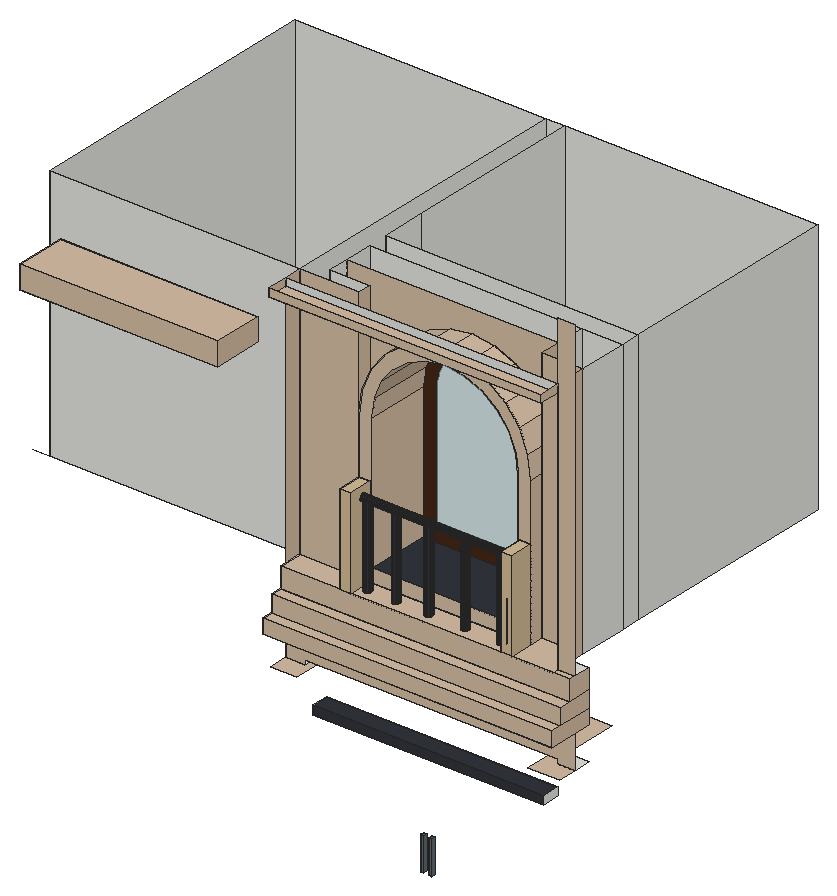
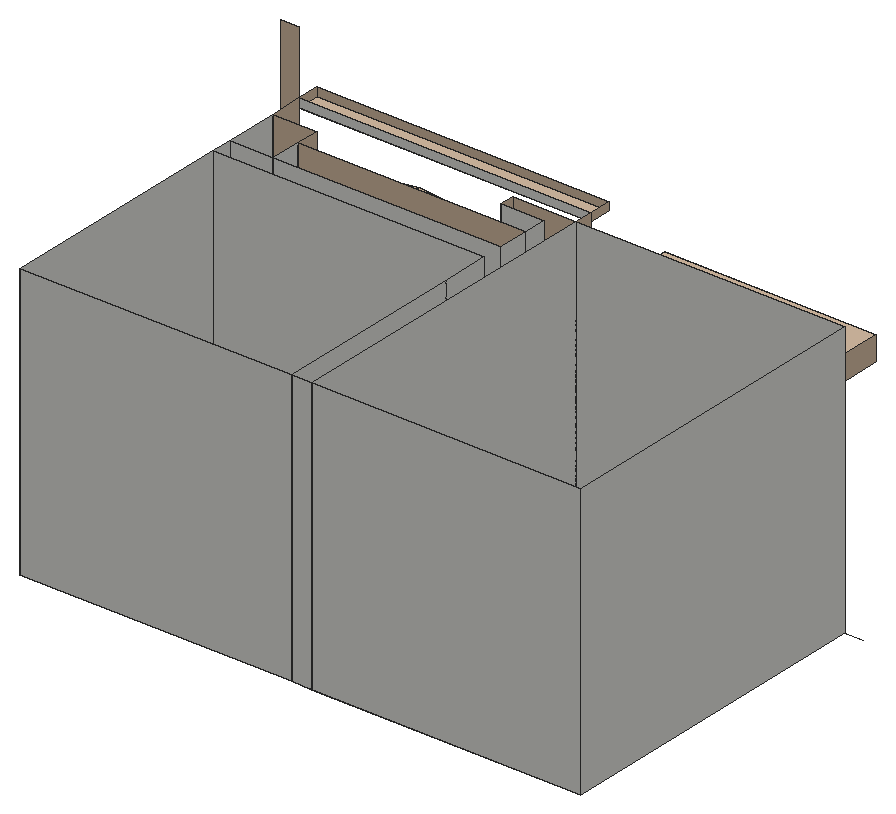
# SketchUp Ruby script. Lengths in inches.
U = 1.inch
M = Sketchup.active_model
def pt(a) = Geom::Point3d.new(a.map { |v| v * U })
def face(e, loops, mat)
  f = e.add_face(loops[0].map { |a| pt(a) })
  loops[1..].each { |l| e.add_face(l.map { |a| pt(a) }).erase! }
  f.material = f.back_material = mat if mat
  f
end
# faces: each face lists its corners as indices into pts; further lists are holes
def faces(e, pts, list, mat = nil) = list.each { |f| face(e, (f[0].is_a?(Array) ? f : [f]).map { |l| l.map { |i| pts[i] } }, mat) }
# xy, xz, yz: faces in a plane at the given z, y or x. An outline is a flat list of corners, or four numbers for a rectangle; further outlines are holes
def ring(l) = l.size == 4 ? [[l[0], l[1]], [l[2], l[1]], [l[2], l[3]], [l[0], l[3]]] : l.each_slice(2).to_a
def flat(e, list, mat, &to3) = list.each { |f| face(e, (f[0].is_a?(Array) ? f : [f]).map { |l| ring(l).map { |u, v| to3.(u, v) } }, mat) }
def xy(e, z, list, mat = nil) = flat(e, list, mat) { |x, y| [x, y, z] }
def xz(e, y, list, mat = nil) = flat(e, list, mat) { |x, z| [x, y, z] }
def yz(e, x, list, mat = nil) = flat(e, list, mat) { |y, z| [x, y, z] }
def lines(e, pts, list) = list.each { |a, b| e.add_line(pt(pts[a]), pt(pts[b])) }
# prism: a flat outline (further loops are holes) pulled along v
def prism(e, loops, v, mat = nil)
  f = face(e, loops, mat); d = Geom::Vector3d.new(v.map { |x| x * U })
  f.pushpull(f.normal.samedirection?(d) ? d.length : -d.length)
end
def box(e, o, s, mat = nil) = prism(e, [[o, [o[0] + s[0], o[1], o[2]], [o[0] + s[0], o[1] + s[1], o[2]], [o[0], o[1] + s[1], o[2]]]], [0, 0, s[2]], mat)
def at(x, y, z, deg = 0) = Geom::Transformation.translation(pt([x, y, z])) * Geom::Transformation.rotation(ORIGIN, Z_AXIS, deg.degrees)
def axes(o, x, y, z) = Geom::Transformation.new([*x, 0, *y, 0, *z, 0, *pt(o).to_a, 1])
def part(name) = M.definitions.add(name)
# library, detail: a bought-in or finely detailed component or shape, given as its bounding box
def library(name, o, s) = part(name).tap { |d| box(d.entities, o, s) }
def detail(e, o, s) = box(e.add_group.entities, o, s)
def put(e, d, t, mat = nil) = e.add_instance(d, t).tap { |i| i.material = mat if mat }
def group(e, t, mat = nil) = e.add_group.tap { |g| g.transformation = t; g.material = mat if mat }.entities
root = M.entities
M.materials.add("[Formica Beige]").color = [211, 187, 149]
M.materials.add("[Formica Laminate Dark]").color = [50, 53, 60]
M.materials.add("[Formica Laminate Light]").color = [213, 189, 164]
M.materials.add("[Formica Speckled Grey]").color = [94, 105, 111]
M.materials.add("[Translucent Glass Safety]").color = [204, 235, 244]
M.materials["[Translucent Glass Safety]"].alpha = 0.5
M.materials.add("[Wood Veneer 01]").color = [68, 40, 21]
xy(root,44.27,[[216.72,67.98,217.85,69.35],[219.85,67.98,220.97,69.35]],"[Formica Speckled Grey]")
xy(root,56.83,[[216.72,67.98,217.85,69.35],[219.85,67.98,220.97,69.35]],"[Formica Speckled Grey]")
xy(root,81.84,[[[175.36,69.35,216.21,75.87],[213.5,71.93,213.76,71.96,214,72.0625,214.21,72.22,214.37,72.43,214.46,72.67,214.5,72.93,214.46,73.1875,214.37,73.43,214.21,73.63,214,73.79,213.76,73.89,213.5,73.93,213.24,73.89,213,73.79,212.79,73.63,212.63,73.43,212.53,73.1875,212.5,72.93,212.53,72.67,212.63,72.43,212.79,72.22,213,72.0625,213.24,71.96],[209.0625,71.93,209.32,71.96,209.5625,72.0625,209.77,72.22,209.93,72.43,210.03,72.67,210.0625,72.93,210.03,73.1875,209.93,73.43,209.77,73.63,209.5625,73.79,209.32,73.89,209.0625,73.93,208.8,73.89,208.5625,73.79,208.35,73.63,208.2,73.43,208.1,73.1875,208.0625,72.93,208.1,72.67,208.2,72.43,208.35,72.22,208.5625,72.0625,208.8,71.96],[204,71.93,204.26,71.96,204.5,72.0625,204.71,72.22,204.87,72.43,204.96,72.67,205,72.93,204.96,73.1875,204.87,73.43,204.71,73.63,204.5,73.79,204.26,73.89,204,73.93,203.74,73.89,203.5,73.79,203.29,73.63,203.13,73.43,203.03,73.1875,203,72.93,203.03,72.67,203.13,72.43,203.29,72.22,203.5,72.0625,203.74,71.96],[199.4375,71.93,199.7,71.96,199.9375,72.0625,200.14,72.22,200.3,72.43,200.4,72.67,200.4375,72.93,200.4,73.1875,200.3,73.43,200.14,73.63,199.9375,73.79,199.7,73.89,199.4375,73.93,199.18,73.89,198.9375,73.79,198.73,73.63,198.57,73.43,198.47,73.1875,198.4375,72.93,198.47,72.67,198.57,72.43,198.73,72.22,198.9375,72.0625,199.18,71.96],[195,71.93,195.26,71.96,195.5,72.0625,195.71,72.22,195.87,72.43,195.96,72.67,196,72.93,195.96,73.1875,195.87,73.43,195.71,73.63,195.5,73.79,195.26,73.89,195,73.93,194.74,73.89,194.5,73.79,194.29,73.63,194.13,73.43,194.03,73.1875,194,72.93,194.03,72.67,194.13,72.43,194.29,72.22,194.5,72.0625,194.74,71.96],[190.75,71.93,191.01,71.96,191.25,72.0625,191.46,72.22,191.62,72.43,191.71,72.67,191.75,72.93,191.71,73.1875,191.62,73.43,191.46,73.63,191.25,73.79,191.01,73.89,190.75,73.93,190.49,73.89,190.25,73.79,190.04,73.63,189.88,73.43,189.78,73.1875,189.75,72.93,189.78,72.67,189.88,72.43,190.04,72.22,190.25,72.0625,190.49,71.96],[186.1875,71.93,186.45,71.96,186.6875,72.0625,186.89,72.22,187.05,72.43,187.15,72.67,187.1875,72.93,187.15,73.1875,187.05,73.43,186.89,73.63,186.6875,73.79,186.45,73.89,186.1875,73.93,185.93,73.89,185.6875,73.79,185.48,73.63,185.32,73.43,185.22,73.1875,185.1875,72.93,185.22,72.67,185.32,72.43,185.48,72.22,185.6875,72.0625,185.93,71.96],[181.5,71.93,181.76,71.96,182,72.0625,182.21,72.22,182.37,72.43,182.46,72.67,182.5,72.93,182.46,73.1875,182.37,73.43,182.21,73.63,182,73.79,181.76,73.89,181.5,73.93,181.24,73.89,181,73.79,180.79,73.63,180.63,73.43,180.53,73.1875,180.5,72.93,180.53,72.67,180.63,72.43,180.79,72.22,181,72.0625,181.24,71.96],[177.5,71.93,177.76,71.96,178,72.0625,178.21,72.22,178.37,72.43,178.46,72.67,178.5,72.93,178.46,73.1875,178.37,73.43,178.21,73.63,178,73.79,177.76,73.89,177.5,73.93,177.24,73.89,177,73.79,176.79,73.63,176.63,73.43,176.53,73.1875,176.5,72.93,176.53,72.67,176.63,72.43,176.79,72.22,177,72.0625,177.24,71.96]],[219.08,69.35,221.95,75.87],[[221.95,69.35,261.51,75.87],[225.25,71.93,225.51,71.96,225.75,72.0625,225.96,72.22,226.12,72.43,226.21,72.67,226.25,72.93,226.21,73.1875,226.12,73.43,225.96,73.63,225.75,73.79,225.51,73.89,225.25,73.93,224.99,73.89,224.75,73.79,224.54,73.63,224.38,73.43,224.28,73.1875,224.25,72.93,224.28,72.67,224.38,72.43,224.54,72.22,224.75,72.0625,224.99,71.96],[229.8125,71.93,230.07,71.96,230.3125,72.0625,230.52,72.22,230.68,72.43,230.78,72.67,230.8125,72.93,230.78,73.1875,230.68,73.43,230.52,73.63,230.3125,73.79,230.07,73.89,229.8125,73.93,229.55,73.89,229.3125,73.79,229.1,73.63,228.95,73.43,228.85,73.1875,228.8125,72.93,228.85,72.67,228.95,72.43,229.1,72.22,229.3125,72.0625,229.55,71.96],[234.1875,71.93,234.45,71.96,234.6875,72.0625,234.89,72.22,235.05,72.43,235.15,72.67,235.1875,72.93,235.15,73.1875,235.05,73.43,234.89,73.63,234.6875,73.79,234.45,73.89,234.1875,73.93,233.93,73.89,233.6875,73.79,233.48,73.63,233.32,73.43,233.22,73.1875,233.1875,72.93,233.22,72.67,233.32,72.43,233.48,72.22,233.6875,72.0625,233.93,71.96],[244.5625,71.93,244.82,71.96,245.0625,72.0625,245.27,72.22,245.43,72.43,245.53,72.67,245.5625,72.93,245.53,73.1875,245.43,73.43,245.27,73.63,245.0625,73.79,244.82,73.89,244.5625,73.93,244.3,73.89,244.0625,73.79,243.85,73.63,243.7,73.43,243.6,73.1875,243.5625,72.93,243.6,72.67,243.7,72.43,243.85,72.22,244.0625,72.0625,244.3,71.96],[249.3125,71.93,249.57,71.96,249.8125,72.0625,250.02,72.22,250.18,72.43,250.28,72.67,250.3125,72.93,250.28,73.1875,250.18,73.43,250.02,73.63,249.8125,73.79,249.57,73.89,249.3125,73.93,249.05,73.89,248.8125,73.79,248.6,73.63,248.45,73.43,248.35,73.1875,248.3125,72.93,248.35,72.67,248.45,72.43,248.6,72.22,248.8125,72.0625,249.05,71.96],[254.25,71.93,254.51,71.96,254.75,72.0625,254.96,72.22,255.12,72.43,255.21,72.67,255.25,72.93,255.21,73.1875,255.12,73.43,254.96,73.63,254.75,73.79,254.51,73.89,254.25,73.93,253.99,73.89,253.75,73.79,253.54,73.63,253.38,73.43,253.28,73.1875,253.25,72.93,253.28,72.67,253.38,72.43,253.54,72.22,253.75,72.0625,253.99,71.96],[239.1875,71.93,239.45,71.96,239.6875,72.0625,239.89,72.22,240.05,72.43,240.15,72.67,240.1875,72.93,240.15,73.1875,240.05,73.43,239.89,73.63,239.6875,73.79,239.45,73.89,239.1875,73.93,238.93,73.89,238.6875,73.79,238.48,73.63,238.32,73.43,238.22,73.1875,238.1875,72.93,238.22,72.67,238.32,72.43,238.48,72.22,238.6875,72.0625,238.93,71.96],[258.6875,71.93,258.95,71.96,259.1875,72.0625,259.39,72.22,259.55,72.43,259.65,72.67,259.6875,72.93,259.65,73.1875,259.55,73.43,259.39,73.63,259.1875,73.79,258.95,73.89,258.6875,73.93,258.43,73.89,258.1875,73.79,257.98,73.63,257.82,73.43,257.72,73.1875,257.6875,72.93,257.72,72.67,257.82,72.43,257.98,72.22,258.1875,72.0625,258.43,71.96]]])
xy(root,84.9,[[175.36,69.35,261.51,75.87]],"[Formica Laminate Dark]")
xy(root,97.5,[[165.35,69.35,172.48,75.87],[266.79,69.35,273.31,75.87]])
xy(root,97.5,[[165.35,61.98,175.36,61.98,175.36,75.87,172.48,75.87,172.48,69.35,165.35,69.35],[261.51,61.98,273.31,61.98,273.31,69.35,266.79,69.35,266.79,75.87,261.51,75.87]],"[Formica Laminate Light]")
xy(root,98.95,[[172.48,69.35,266.79,94.48]],"[Formica Laminate Light]")
xy(root,109.89,[[165.35,69.35,273.31,75.87]])
xy(root,109.89,[[165.35,58.62,273.31,69.35]],"[Formica Laminate Light]")
xy(root,115.3,[[165.35,62.49,273.31,75.87]])
xy(root,115.3,[[165.35,58.62,273.31,62.49]],"[Formica Laminate Light]")
xy(root,121.5,[[165.35,66.99,273.31,75.87]])
xy(root,121.5,[[165.35,62.49,273.31,66.99]],"[Formica Laminate Light]")
xy(root,129,[[187.4,66.99,191.47,75.87],[247.3,66.99,251.59,75.87],[266.79,69.35,273.31,75.87],[194.31,69.95,193.95,70,193.62,70.14,193.34,70.36,193.12,70.64,192.98,70.97,192.94,71.33,192.98,71.68,193.12,72.02,193.34,72.3,193.62,72.52,193.95,72.66,194.31,72.7,194.67,72.66,195,72.52,195.28,72.3,195.5,72.02,195.64,71.68,195.69,71.33,195.64,70.97,195.5,70.64,195.28,70.36,195,70.14,194.67,70],[204.81,69.95,204.45,70,204.12,70.14,203.84,70.36,203.62,70.64,203.48,70.97,203.44,71.33,203.48,71.68,203.62,72.02,203.84,72.3,204.12,72.52,204.45,72.66,204.81,72.7,205.17,72.66,205.5,72.52,205.78,72.3,206,72.02,206.14,71.68,206.19,71.33,206.14,70.97,206,70.64,205.78,70.36,205.5,70.14,205.17,70],
  [217.06,69.95,216.7,70,216.37,70.14,216.09,70.36,215.87,70.64,215.73,70.97,215.69,71.33,215.73,71.68,215.87,72.02,216.09,72.3,216.37,72.52,216.7,72.66,217.06,72.7,217.42,72.66,217.75,72.52,218.03,72.3,218.25,72.02,218.39,71.68,218.44,71.33,218.39,70.97,218.25,70.64,218.03,70.36,217.75,70.14,217.42,70],[230.69,69.95,230.33,70,230,70.14,229.71,70.36,229.49,70.64,229.36,70.97,229.31,71.33,229.36,71.68,229.49,72.02,229.71,72.3,230,72.52,230.33,72.66,230.69,72.7,231.04,72.66,231.37,72.52,231.66,72.3,231.875,72.02,232.01,71.68,232.06,71.33,232.01,70.97,231.875,70.64,231.66,70.36,231.37,70.14,231.04,70],[244.31,69.95,243.95,70,243.62,70.14,243.34,70.36,243.12,70.64,242.98,70.97,242.94,71.33,242.98,71.68,243.12,72.02,243.34,72.3,243.62,72.52,243.95,72.66,244.31,72.7,244.67,72.66,245,72.52,245.28,72.3,245.5,72.02,245.64,71.68,245.69,71.33,245.64,70.97,245.5,70.64,245.28,70.36,245,70.14,244.67,70],[71.76,75.87,165.35,190.6],[165.35,75.87,172.48,75.87,172.48,99.67,266.79,99.67,266.79,106.73,172.48,106.73,172.48,190.6,165.35,190.6],
  [187.4,75.87,251.59,80.84],[172.48,80.84,187.4,88.8],[187.4,80.84,251.59,99.67],[172.48,88.8,187.4,99.67],[172.48,106.73,266.79,190.6]])
xy(root,129,[[165.35,66.99,187.4,75.87],[[191.47,66.99,247.3,75.87],[244.31,69.95,243.95,70,243.62,70.14,243.34,70.36,243.12,70.64,242.98,70.97,242.94,71.33,242.98,71.68,243.12,72.02,243.34,72.3,243.62,72.52,243.95,72.66,244.31,72.7,244.67,72.66,245,72.52,245.28,72.3,245.5,72.02,245.64,71.68,245.69,71.33,245.64,70.97,245.5,70.64,245.28,70.36,245,70.14,244.67,70],[194.31,69.95,193.95,70,193.62,70.14,193.34,70.36,193.12,70.64,192.98,70.97,192.94,71.33,192.98,71.68,193.12,72.02,193.34,72.3,193.62,72.52,193.95,72.66,194.31,72.7,194.67,72.66,195,72.52,195.28,72.3,195.5,72.02,195.64,71.68,195.69,71.33,195.64,70.97,195.5,70.64,195.28,70.36,195,70.14,194.67,70],[230.69,69.95,230.33,70,230,70.14,229.71,70.36,229.49,70.64,229.36,70.97,229.31,71.33,229.36,71.68,229.49,72.02,229.71,72.3,230,72.52,230.33,72.66,230.69,72.7,231.04,72.66,231.37,72.52,231.66,72.3,231.875,72.02,232.01,71.68,232.06,71.33,232.01,70.97,231.875,70.64,231.66,70.36,231.37,70.14,231.04,70],[204.81,69.95,204.45,70,204.12,70.14,203.84,70.36,203.62,70.64,203.48,70.97,203.44,71.33,203.48,71.68,203.62,72.02,203.84,72.3,204.12,72.52,204.45,72.66,204.81,72.7,205.17,72.66,205.5,72.52,205.78,72.3,206,72.02,206.14,71.68,206.19,71.33,206.14,70.97,206,70.64,205.78,70.36,205.5,70.14,205.17,70],[217.06,69.95,216.7,70,216.37,70.14,216.09,70.36,215.87,70.64,215.73,70.97,215.69,71.33,215.73,71.68,215.87,72.02,216.09,72.3,216.37,72.52,216.7,72.66,217.06,72.7,217.42,72.66,217.75,72.52,218.03,72.3,218.25,72.02,218.39,71.68,218.44,71.33,218.39,70.97,218.25,70.64,218.03,70.36,217.75,70.14,217.42,70]],[251.59,66.99,266.79,80.84],[266.79,66.99,273.31,69.35]],"[Formica Laminate Light]")
xy(root,133.77,[[192.17,75.87,246.82,99.67]],"[Formica Laminate Dark]")
xy(root,158.75,[[204.81,69.95,205.17,70,205.5,70.14,205.78,70.36,206,70.64,206.14,70.97,206.19,71.33,206.14,71.68,206,72.02,205.78,72.3,205.5,72.52,205.17,72.66,204.81,72.7,204.45,72.66,204.12,72.52,203.84,72.3,203.62,72.02,203.48,71.68,203.44,71.33,203.48,70.97,203.62,70.64,203.84,70.36,204.12,70.14,204.45,70]])
xy(root,159.125,[[194.31,69.95,194.67,70,195,70.14,195.28,70.36,195.5,70.64,195.64,70.97,195.69,71.33,195.64,71.68,195.5,72.02,195.28,72.3,195,72.52,194.67,72.66,194.31,72.7,193.95,72.66,193.62,72.52,193.34,72.3,193.12,72.02,192.98,71.68,192.94,71.33,192.98,70.97,193.12,70.64,193.34,70.36,193.62,70.14,193.95,70]])
xy(root,159.1875,[[244.31,69.95,244.67,70,245,70.14,245.28,70.36,245.5,70.64,245.64,70.97,245.69,71.33,245.64,71.68,245.5,72.02,245.28,72.3,245,72.52,244.67,72.66,244.31,72.7,243.95,72.66,243.62,72.52,243.34,72.3,243.12,72.02,242.98,71.68,242.94,71.33,242.98,70.97,243.12,70.64,243.34,70.36,243.62,70.14,243.95,70]])
xy(root,159.5625,[[217.06,69.95,217.42,70,217.75,70.14,218.03,70.36,218.25,70.64,218.39,70.97,218.44,71.33,218.39,71.68,218.25,72.02,218.03,72.3,217.75,72.52,217.42,72.66,217.06,72.7,216.7,72.66,216.37,72.52,216.09,72.3,215.87,72.02,215.73,71.68,215.69,71.33,215.73,70.97,215.87,70.64,216.09,70.36,216.37,70.14,216.7,70]])
xy(root,159.625,[[230.69,69.95,231.04,70,231.37,70.14,231.66,70.36,231.875,70.64,232.01,70.97,232.06,71.33,232.01,71.68,231.875,72.02,231.66,72.3,231.37,72.52,231.04,72.66,230.69,72.7,230.33,72.66,230,72.52,229.71,72.3,229.49,72.02,229.36,71.68,229.31,71.33,229.36,70.97,229.49,70.64,229.71,70.36,230,70.14,230.33,70]])
xy(root,162.625,[[187.4,66.99,191.47,75.87],[247.3,66.99,251.59,75.87]],"[Formica Beige]")
xy(root,199.15,[[87.96,59.04,144.31,69.35]])
xy(root,199.15,[[81.08,50.48,81.08,69.35,87.96,69.35,87.96,59.04,144.31,59.04,144.31,69.35,154.75,69.35,154.75,50.48]],"[Formica Laminate Light]")
xy(root,207.68,[[81.08,50.48,154.75,69.35]],"[Formica Laminate Light]")
xy(root,221.5,[[165.35,61.48,266.79,69.35]],"[Formica Laminate Light]")
xz(root,50.48,[[81.08,199.15,154.75,207.68]],"[Formica Laminate Light]")
xz(root,58.62,[[165.35,109.89,273.31,115.3]],"[Formica Laminate Light]")
xz(root,61.48,[[165.35,221.5,266.79,224.375]],"[Formica Laminate Light]")
xz(root,62.49,[[165.35,115.3,273.31,121.5]],"[Formica Laminate Light]")
xz(root,66.99,[[187.4,129,191.47,162.625],[247.3,129,251.59,162.625]],"[Formica Beige]")
xz(root,66.99,[[165.35,121.5,273.31,129]],"[Formica Laminate Light]")
xz(root,67.98,[[216.72,44.27,217.85,56.83],[219.85,44.27,220.97,56.83]],"[Formica Speckled Grey]")
xz(root,69.35,[[81.08,199.15,154.75,207.68],[165.35,221.5,266.79,224.375]])
xz(root,69.35,[[175.36,81.84,261.51,84.9]],"[Formica Laminate Dark]")
xz(root,69.35,[[165.35,97.5,172.48,97.5,172.48,98.95,266.79,98.95,266.79,97.5,273.31,97.5,273.31,109.89,165.35,109.89],[266.79,129,273.31,246.5]],"[Formica Laminate Light]")
xz(root,75.87,[[175.36,81.84,261.51,84.9],[165.35,109.89,273.31,115.3],[165.35,115.3,273.31,121.5],[71.76,129,165.35,224.375],[187.4,129,191.47,162.625],
  [247.3,129,251.59,162.625]])
xz(root,75.87,[[165.35,129,187.4,224.375],[[191.47,129,247.3,129,247.3,162.625,251.59,162.625,251.59,183.9375,250.5,192.24,247.29,199.98,242.1875,206.63,235.54,211.73,227.8,214.9375,219.49,216.03,211.1875,214.9375,203.45,211.73,196.8,206.63,191.7,199.98,188.49,192.24,187.4,183.9375,187.4,162.625,191.47,162.625],[192.17,133.77,192.17,183.9375,193.1,191.01,195.83,197.6,200.17,203.26,205.83,207.6,212.42,210.33,219.49,211.27,226.57,210.33,233.16,207.6,238.82,203.26,243.16,197.6,245.89,191.01,246.82,183.9375,246.82,133.77]]],"[Formica Laminate Light]")
xz(root,80.84,[[172.48,129,187.4,224.375]])
xz(root,80.84,[[251.59,129,266.79,224.375]],"[Formica Laminate Light]")
xz(root,88.8,[[172.48,129,187.4,129,187.4,183.9375,188.49,192.24,191.7,199.98,196.8,206.63,203.45,211.73,211.1875,214.9375,219.49,216.03,227.8,214.9375,235.54,211.73,242.1875,206.63,247.29,199.98,250.5,192.24,251.59,183.9375,251.59,224.375,172.48,224.375]],"[Formica Laminate Light]")
xz(root,99.67,[[172.48,129,172.48,224.375,251.59,224.375,251.59,183.9375,250.5,192.24,247.29,199.98,242.1875,206.63,235.54,211.73,227.8,214.9375,219.49,216.03,211.1875,214.9375,203.45,211.73,196.8,206.63,191.7,199.98,188.49,192.24,187.4,183.9375,187.4,129],[251.59,129,266.79,224.375]])
xz(root,99.67,[[197.19,138.79,241.8,138.79,241.8,183.9375,241.77,185.1,241.68,186.27,241.52,187.43,241.3125,188.57,241.04,189.71,240.71,190.83,240.32,191.93,239.87,193.01,239.37,194.0625,238.8125,195.09,238.2,196.09,237.54,197.05,236.83,197.97,236.07,198.86,235.27,199.71,234.42,200.51,233.53,201.27,232.6,201.98,231.64,202.64,230.65,203.25,229.62,203.8125,228.57,204.3125,227.49,204.76,226.39,205.15,225.27,205.48,224.13,205.75,222.98,205.97,221.83,206.12,220.66,206.21,219.49,206.24,218.33,206.21,217.16,206.12,216.01,205.97,214.86,205.75,213.72,205.48,212.6,205.15,211.5,204.76,210.42,204.3125,209.37,203.8125,208.34,203.25,207.35,202.64,206.38,201.98,205.46,201.27,204.57,200.51,203.72,199.71,202.92,198.86,202.16,197.97,201.45,197.05,200.79,196.09,200.18,195.09,199.62,194.0625,199.12,193.01,198.67,191.93,198.28,190.83,197.95,189.71,197.68,188.57,197.47,187.43,197.3125,186.27,197.22,185.1,197.19,183.9375]],"[Translucent Glass Safety]")
xz(root,99.67,[[[192.17,133.77,246.82,133.77,246.82,183.9375,245.89,191.01,243.16,197.6,238.82,203.26,233.16,207.6,226.57,210.33,219.49,211.27,212.42,210.33,205.83,207.6,200.17,203.26,195.83,197.6,193.1,191.01,192.17,183.9375],[197.19,138.79,197.19,183.9375,197.22,185.1,197.3125,186.27,197.47,187.43,197.68,188.57,197.95,189.71,198.28,190.83,198.67,191.93,199.12,193.01,199.62,194.0625,200.18,195.09,200.79,196.09,201.45,197.05,202.16,197.97,202.92,198.86,203.72,199.71,204.57,200.51,205.46,201.27,206.38,201.98,207.35,202.64,208.34,203.25,209.37,203.8125,210.42,204.3125,211.5,204.76,212.6,205.15,213.72,205.48,214.86,205.75,216.01,205.97,217.16,206.12,218.33,206.21,219.49,206.24,220.66,206.21,221.83,206.12,222.98,205.97,224.13,205.75,225.27,205.48,226.39,205.15,227.49,204.76,228.57,204.3125,229.62,203.8125,230.65,203.25,231.64,202.64,232.6,201.98,233.53,201.27,234.42,200.51,235.27,199.71,236.07,198.86,236.83,197.97,237.54,197.05,238.2,196.09,238.8125,195.09,239.37,194.0625,239.87,193.01,240.32,191.93,240.71,190.83,241.04,189.71,241.3125,188.57,241.52,187.43,241.68,186.27,241.77,185.1,241.8,183.9375,241.8,138.79]]],"[Wood Veneer 01]")
xz(root,106.73,[[172.48,129,266.79,224.375]])
xz(root,190.6,[[71.76,129,165.35,224.375],[165.35,129,172.48,224.375],[172.48,129,266.79,224.375]])
yz(root,71.76,[[75.87,129,190.6,224.375]])
yz(root,81.08,[[50.48,199.15,69.35,207.68]],"[Formica Laminate Light]")
yz(root,154.75,[[50.48,199.15,69.35,207.68]],"[Formica Laminate Light]")
yz(root,165.35,[[69.35,97.5,75.87,109.89],[69.35,109.89,75.87,115.3],[69.35,115.3,75.87,121.5],[69.35,121.5,75.87,129],[75.87,129,190.6,224.375]])
yz(root,165.35,[[58.62,109.89,69.35,115.3],[62.49,115.3,69.35,121.5],[66.99,121.5,69.35,129],[69.35,129,75.87,224.375],[61.48,221.5,69.35,224.375]],"[Formica Laminate Light]")
yz(root,172.48,[[80.84,129,88.8,224.375],[88.8,129,99.67,224.375],[106.73,129,123.48,224.375],[123.48,129,190.6,224.375]])
yz(root,175.36,[[69.35,81.84,75.87,84.9]])
yz(root,187.4,[[75.87,129,80.84,183.9375],[80.84,129,88.8,183.9375],[88.8,129,99.67,183.9375]])
yz(root,187.4,[[66.99,129,75.87,162.625]],"[Formica Beige]")
yz(root,187.4,[[75.87,183.9375,80.84,224.375]],"[Formica Laminate Light]")
yz(root,191.47,[[[66.99,129,75.87,162.625],[72,157.91,71.7,157.95,71.41,158.07,71.16,158.26,70.98,158.51,70.86,158.79,70.82,159.1,70.86,159.41,70.98,159.69,71.16,159.9375,71.41,160.13,71.7,160.25,72,160.29,72.3125,160.25,72.6,160.13,72.84,159.9375,73.03,159.69,73.15,159.41,73.19,159.1,73.15,158.79,73.03,158.51,72.84,158.26,72.6,158.07,72.3125,157.95]]],"[Formica Beige]")
yz(root,192.17,[[75.87,133.77,99.67,183.9375]],"[Formica Laminate Light]")
yz(root,216.72,[[67.98,44.27,69.35,56.83]],"[Formica Speckled Grey]")
yz(root,217.85,[[67.98,44.27,69.35,56.83]],"[Formica Speckled Grey]")
yz(root,219.85,[[67.98,44.27,69.35,56.83]],"[Formica Speckled Grey]")
yz(root,220.97,[[67.98,44.27,69.35,56.83]],"[Formica Speckled Grey]")
yz(root,246.82,[[75.87,133.77,99.67,183.9375]],"[Formica Laminate Light]")
yz(root,247.3,[[72,157.91,72.3125,157.95,72.6,158.07,72.84,158.26,73.03,158.51,73.15,158.79,73.19,159.1,73.15,159.41,73.03,159.69,72.84,159.9375,72.6,160.13,72.3125,160.25,72,160.29,71.7,160.25,71.41,160.13,71.16,159.9375,70.98,159.69,70.86,159.41,70.82,159.1,70.86,158.79,70.98,158.51,71.16,158.26,71.41,158.07,71.7,157.95]])
yz(root,247.3,[[[66.99,129,75.87,162.625],[72,157.91,72.3125,157.95,72.6,158.07,72.84,158.26,73.03,158.51,73.15,158.79,73.19,159.1,73.15,159.41,73.03,159.69,72.84,159.9375,72.6,160.13,72.3125,160.25,72,160.29,71.7,160.25,71.41,160.13,71.16,159.9375,70.98,159.69,70.86,159.41,70.82,159.1,70.86,158.79,70.98,158.51,71.16,158.26,71.41,158.07,71.7,157.95]]],"[Formica Beige]")
yz(root,251.59,[[80.84,129,99.67,183.9375],[88.8,183.9375,99.67,224.375]])
yz(root,251.59,[[66.99,129,75.87,162.625]],"[Formica Beige]")
yz(root,251.59,[[75.87,129,80.84,183.9375],[80.84,183.9375,88.8,224.375]],"[Formica Laminate Light]")
yz(root,261.51,[[69.35,81.84,75.87,84.9]])
yz(root,266.79,[[80.84,129,99.67,224.375],[99.67,129,106.73,224.375],[106.73,129,190.6,224.375]])
yz(root,266.79,[[69.35,129,80.84,224.375],[61.48,221.5,69.35,224.375]],"[Formica Laminate Light]")
yz(root,273.31,[[58.62,109.89,75.87,115.3],[62.49,115.3,75.87,121.5],[66.99,121.5,75.87,129]],"[Formica Laminate Light]")
p = [[193.62,70.14,129],[193.95,70,129],[193.95,70,159.125],[193.62,70.14,159.125],[194.31,69.95,129],[194.31,69.95,159.125],
  [194.67,70,129],[194.67,70,159.125],[195,70.14,129],[195,70.14,159.125],[204.12,70.14,129],[204.45,70,129],
  [204.45,70,158.75],[204.12,70.14,158.75],[204.81,69.95,129],[204.81,69.95,158.75],[205.17,70,129],[205.17,70,158.75],
  [205.5,70.14,129],[205.5,70.14,158.75],[216.37,70.14,129],[216.7,70,129],[216.7,70,159.5625],[216.37,70.14,159.5625],
  [217.06,69.95,129],[217.06,69.95,159.5625],[217.42,70,129],[217.42,70,159.5625],[217.75,70.14,129],[217.75,70.14,159.5625],
  [230,70.14,129],[230.33,70,129],[230.33,70,159.625],[230,70.14,159.625],[230.69,69.95,129],[230.69,69.95,159.625],
  [231.04,70,129],[231.04,70,159.625],[231.37,70.14,129],[231.37,70.14,159.625],[243.62,70.14,129],[243.95,70,129],
  [243.95,70,159.1875],[243.62,70.14,159.1875],[244.31,69.95,129],[244.31,69.95,159.1875],[244.67,70,129],[244.67,70,159.1875],
  [245,70.14,129],[245,70.14,159.1875],[193.34,70.36,129],[193.34,70.36,159.125],[195.28,70.36,129],[195.28,70.36,159.125],
  [203.84,70.36,129],[203.84,70.36,158.75],[205.78,70.36,129],[205.78,70.36,158.75],[216.09,70.36,129],[216.09,70.36,159.5625],
  [218.03,70.36,129],[218.03,70.36,159.5625],[229.71,70.36,129],[229.71,70.36,159.625],[231.66,70.36,129],[231.66,70.36,159.625],
  [243.34,70.36,129],[243.34,70.36,159.1875],[245.28,70.36,129],[245.28,70.36,159.1875],[193.12,70.64,129],[193.12,70.64,159.125],
  [195.5,70.64,129],[195.5,70.64,159.125],[203.62,70.64,129],[203.62,70.64,158.75],[206,70.64,129],[206,70.64,158.75],
  [215.87,70.64,129],[215.87,70.64,159.5625],[218.25,70.64,129],[218.25,70.64,159.5625],[229.49,70.64,129],[229.49,70.64,159.625],
  [231.875,70.64,129],[231.875,70.64,159.625],[243.12,70.64,129],[243.12,70.64,159.1875],[245.5,70.64,129],[245.5,70.64,159.1875],
  [192.98,70.97,129],[192.98,70.97,159.125],[195.64,70.97,129],[195.64,70.97,159.125],[203.48,70.97,129],[203.48,70.97,158.75],
  [206.14,70.97,129],[206.14,70.97,158.75],[215.73,70.97,129],[215.73,70.97,159.5625],[218.39,70.97,129],[218.39,70.97,159.5625],
  [229.36,70.97,129],[229.36,70.97,159.625],[232.01,70.97,129],[232.01,70.97,159.625],[242.98,70.97,129],[242.98,70.97,159.1875],
  [245.64,70.97,129],[245.64,70.97,159.1875],[192.94,71.33,129],[192.94,71.33,159.125],[195.69,71.33,129],[195.69,71.33,159.125],
  [203.44,71.33,129],[203.44,71.33,158.75],[206.19,71.33,129],[206.19,71.33,158.75],[215.69,71.33,129],[215.69,71.33,159.5625],
  [218.44,71.33,129],[218.44,71.33,159.5625],[229.31,71.33,129],[229.31,71.33,159.625],[232.06,71.33,129],[232.06,71.33,159.625],
  [242.94,71.33,129],[242.94,71.33,159.1875],[245.69,71.33,129],[245.69,71.33,159.1875],[192.98,71.68,129],[192.98,71.68,159.125],
  [195.64,71.68,129],[195.64,71.68,159.125],[203.48,71.68,129],[203.48,71.68,158.75],[206.14,71.68,129],[206.14,71.68,158.75],
  [215.73,71.68,129],[215.73,71.68,159.5625],[218.39,71.68,129],[218.39,71.68,159.5625],[229.36,71.68,129],[229.36,71.68,159.625],
  [232.01,71.68,129],[232.01,71.68,159.625],[242.98,71.68,129],[242.98,71.68,159.1875],[245.64,71.68,129],[245.64,71.68,159.1875],
  [193.12,72.02,129],[193.12,72.02,159.125],[195.5,72.02,129],[195.5,72.02,159.125],[203.62,72.02,129],[203.62,72.02,158.75],
  [206,72.02,129],[206,72.02,158.75],[215.87,72.02,129],[215.87,72.02,159.5625],[218.25,72.02,129],[218.25,72.02,159.5625],
  [229.49,72.02,129],[229.49,72.02,159.625],[231.875,72.02,129],[231.875,72.02,159.625],[243.12,72.02,129],[243.12,72.02,159.1875],
  [245.5,72.02,129],[245.5,72.02,159.1875],[193.34,72.3,129],[193.34,72.3,159.125],[195.28,72.3,129],[195.28,72.3,159.125],
  [203.84,72.3,129],[203.84,72.3,158.75],[205.78,72.3,129],[205.78,72.3,158.75],[216.09,72.3,129],[216.09,72.3,159.5625],
  [218.03,72.3,129],[218.03,72.3,159.5625],[229.71,72.3,129],[229.71,72.3,159.625],[231.66,72.3,129],[231.66,72.3,159.625],
  [243.34,72.3,129],[243.34,72.3,159.1875],[245.28,72.3,129],[245.28,72.3,159.1875],[193.62,72.52,129],[193.62,72.52,159.125],
  [195,72.52,129],[195,72.52,159.125],[204.12,72.52,129],[204.12,72.52,158.75],[205.5,72.52,129],[205.5,72.52,158.75],
  [216.37,72.52,129],[216.37,72.52,159.5625],[217.75,72.52,129],[217.75,72.52,159.5625],[230,72.52,129],[230,72.52,159.625],
  [231.37,72.52,129],[231.37,72.52,159.625],[243.62,72.52,129],[243.62,72.52,159.1875],[245,72.52,129],[245,72.52,159.1875],
  [193.95,72.66,129],[193.95,72.66,159.125],[194.67,72.66,129],[194.67,72.66,159.125],[204.45,72.66,129],[204.45,72.66,158.75],
  [205.17,72.66,129],[205.17,72.66,158.75],[216.7,72.66,129],[216.7,72.66,159.5625],[217.42,72.66,129],[217.42,72.66,159.5625],
  [230.33,72.66,129],[230.33,72.66,159.625],[231.04,72.66,129],[231.04,72.66,159.625],[243.95,72.66,129],[243.95,72.66,159.1875],
  [244.67,72.66,129],[244.67,72.66,159.1875],[194.31,72.7,129],[194.31,72.7,159.125],[204.81,72.7,129],[204.81,72.7,158.75],
  [217.06,72.7,129],[217.06,72.7,159.5625],[230.69,72.7,129],[230.69,72.7,159.625],[244.31,72.7,129],[244.31,72.7,159.1875],
  [247.3,72,157.91],[247.3,71.7,157.95],[191.47,71.7,157.95],[191.47,72,157.91],[247.3,72.3125,157.95],[191.47,72.3125,157.95],
  [247.3,71.41,158.07],[191.47,71.41,158.07],[247.3,72.6,158.07],[191.47,72.6,158.07],[247.3,71.16,158.26],[191.47,71.16,158.26],
  [247.3,72.84,158.26],[191.47,72.84,158.26],[247.3,70.98,158.51],[191.47,70.98,158.51],[247.3,73.03,158.51],[191.47,73.03,158.51],
  [247.3,70.86,158.79],[191.47,70.86,158.79],[247.3,73.15,158.79],[191.47,73.15,158.79],[247.3,70.82,159.1],[191.47,70.82,159.1],
  [247.3,73.19,159.1],[191.47,73.19,159.1],[247.3,70.86,159.41],[191.47,70.86,159.41],[247.3,73.15,159.41],[191.47,73.15,159.41],
  [247.3,70.98,159.69],[191.47,70.98,159.69],[247.3,73.03,159.69],[191.47,73.03,159.69],[247.3,71.16,159.9375],[191.47,71.16,159.9375],
  [247.3,72.84,159.9375],[191.47,72.84,159.9375],[247.3,71.41,160.13],[191.47,71.41,160.13],[247.3,72.6,160.13],[191.47,72.6,160.13],
  [247.3,71.7,160.25],[191.47,71.7,160.25],[247.3,72.3125,160.25],[191.47,72.3125,160.25],[247.3,72,160.29],[191.47,72,160.29],
  [188.49,75.87,192.24],[188.49,88.8,192.24],[187.4,88.8,183.9375],[187.4,80.84,183.9375],[187.4,75.87,183.9375],[192.17,99.67,183.9375],
  [193.1,99.67,191.01],[193.1,75.87,191.01],[192.17,75.87,183.9375],[245.89,99.67,191.01],[246.82,99.67,183.9375],[246.82,75.87,183.9375],
  [245.89,75.87,191.01],[251.59,80.84,183.9375],[251.59,88.8,183.9375],[250.5,88.8,192.24],[250.5,75.87,192.24],[251.59,75.87,183.9375],
  [188.49,99.67,192.24],[187.4,99.67,183.9375],[251.59,99.67,183.9375],[250.5,99.67,192.24],[195.83,99.67,197.6],[195.83,75.87,197.6],
  [243.16,99.67,197.6],[243.16,75.87,197.6],[191.7,75.87,199.98],[191.7,88.8,199.98],[247.29,88.8,199.98],[247.29,75.87,199.98],
  [191.7,99.67,199.98],[247.29,99.67,199.98],[200.17,99.67,203.26],[200.17,75.87,203.26],[238.82,99.67,203.26],[238.82,75.87,203.26],
  [196.8,75.87,206.63],[196.8,88.8,206.63],[242.1875,88.8,206.63],[242.1875,75.87,206.63],[196.8,99.67,206.63],[242.1875,99.67,206.63],
  [205.83,99.67,207.6],[205.83,75.87,207.6],[233.16,99.67,207.6],[233.16,75.87,207.6],[203.45,75.87,211.73],[203.45,88.8,211.73],
  [235.54,88.8,211.73],[235.54,75.87,211.73],[203.45,99.67,211.73],[235.54,99.67,211.73],[212.42,99.67,210.33],[212.42,75.87,210.33],
  [226.57,99.67,210.33],[226.57,75.87,210.33],[219.49,99.67,211.27],[219.49,75.87,211.27],[211.1875,75.87,214.9375],[211.1875,88.8,214.9375],
  [227.8,88.8,214.9375],[227.8,75.87,214.9375],[211.1875,99.67,214.9375],[227.8,99.67,214.9375],[219.49,75.87,216.03],[219.49,88.8,216.03],
  [219.49,99.67,216.03],[71.76,75.87,129],[65.24,75.87,129]]
faces(root,p,[[0,1,2,3],[1,4,5,2],[4,6,7,5],[6,8,9,7],[10,11,12,13],[11,14,15,12],[14,16,17,15],[16,18,19,17],
  [20,21,22,23],[21,24,25,22],[24,26,27,25],[26,28,29,27],[30,31,32,33],[31,34,35,32],[34,36,37,35],[36,38,39,37],
  [40,41,42,43],[41,44,45,42],[44,46,47,45],[46,48,49,47],[50,0,3,51],[8,52,53,9],[54,10,13,55],[18,56,57,19],
  [58,20,23,59],[28,60,61,29],[62,30,33,63],[38,64,65,39],[66,40,43,67],[48,68,69,49],[70,50,51,71],[52,72,73,53],
  [74,54,55,75],[56,76,77,57],[78,58,59,79],[60,80,81,61],[82,62,63,83],[64,84,85,65],[86,66,67,87],[68,88,89,69],
  [90,70,71,91],[72,92,93,73],[94,74,75,95],[76,96,97,77],[98,78,79,99],[80,100,101,81],[102,82,83,103],[84,104,105,85],
  [106,86,87,107],[88,108,109,89],[110,90,91,111],[92,112,113,93],[114,94,95,115],[96,116,117,97],[118,98,99,119],[100,120,121,101],
  [122,102,103,123],[104,124,125,105],[126,106,107,127],[108,128,129,109],[130,110,111,131],[112,132,133,113],[134,114,115,135],[116,136,137,117],
  [138,118,119,139],[120,140,141,121],[142,122,123,143],[124,144,145,125],[146,126,127,147],[128,148,149,129],[150,130,131,151],[132,152,153,133],
  [154,134,135,155],[136,156,157,137],[158,138,139,159],[140,160,161,141],[162,142,143,163],[144,164,165,145],[166,146,147,167],[148,168,169,149],
  [170,150,151,171],[152,172,173,153],[174,154,155,175],[156,176,177,157],[178,158,159,179],[160,180,181,161],[182,162,163,183],[164,184,185,165],
  [186,166,167,187],[168,188,189,169],[190,170,171,191],[172,192,193,173],[194,174,175,195],[176,196,197,177],[198,178,179,199],[180,200,201,181],
  [202,182,183,203],[184,204,205,185],[206,186,187,207],[188,208,209,189],[210,190,191,211],[192,212,213,193],[214,194,195,215],[196,216,217,197],
  [218,198,199,219],[200,220,221,201],[222,202,203,223],[204,224,225,205],[226,206,207,227],[208,228,229,209],[230,210,211,231],[212,230,231,213],
  [232,214,215,233],[216,232,233,217],[234,218,219,235],[220,234,235,221],[236,222,223,237],[224,236,237,225],[238,226,227,239],[228,238,239,229],
  [240,241,242,243],[244,240,243,245],[241,246,247,242],[248,244,245,249],[246,250,251,247],[252,248,249,253],[250,254,255,251],[256,252,253,257],
  [254,258,259,255],[260,256,257,261],[258,262,263,259],[264,260,261,265],[262,266,267,263],[268,264,265,269],[266,270,271,267],[272,268,269,273],
  [270,274,275,271],[276,272,273,277],[274,278,279,275],[280,276,277,281],[278,282,283,279],[284,280,281,285],[282,286,287,283],[286,284,285,287]],"[Formica Laminate Dark]")
faces(root,p,[[288,289,290,291,292],[293,294,295,296],[297,298,299,300],[301,302,303,304,305],[294,310,311,295],[312,297,300,313],[314,315,289,288],[304,303,316,317],
  [310,320,321,311],[322,312,313,323],[324,325,315,314],[317,316,326,327],[320,330,331,321],[332,322,323,333],[334,335,325,324],[327,326,336,337],
  [330,340,341,331],[342,332,333,343],[340,344,345,341],[344,342,343,345],[346,347,335,334],[337,336,348,349],[352,353,347,346],[349,348,353,352]],"[Formica Laminate Light]")
faces(root,p,[[306,307,290,289],[308,309,303,302],[318,306,289,315],[309,319,316,303],[328,318,315,325],[319,329,326,316],[338,328,325,335],[329,339,336,326],
  [350,338,335,347],[339,351,348,336],[354,350,347,353],[351,354,353,348]])
lines(root,p,[[355,356]])
